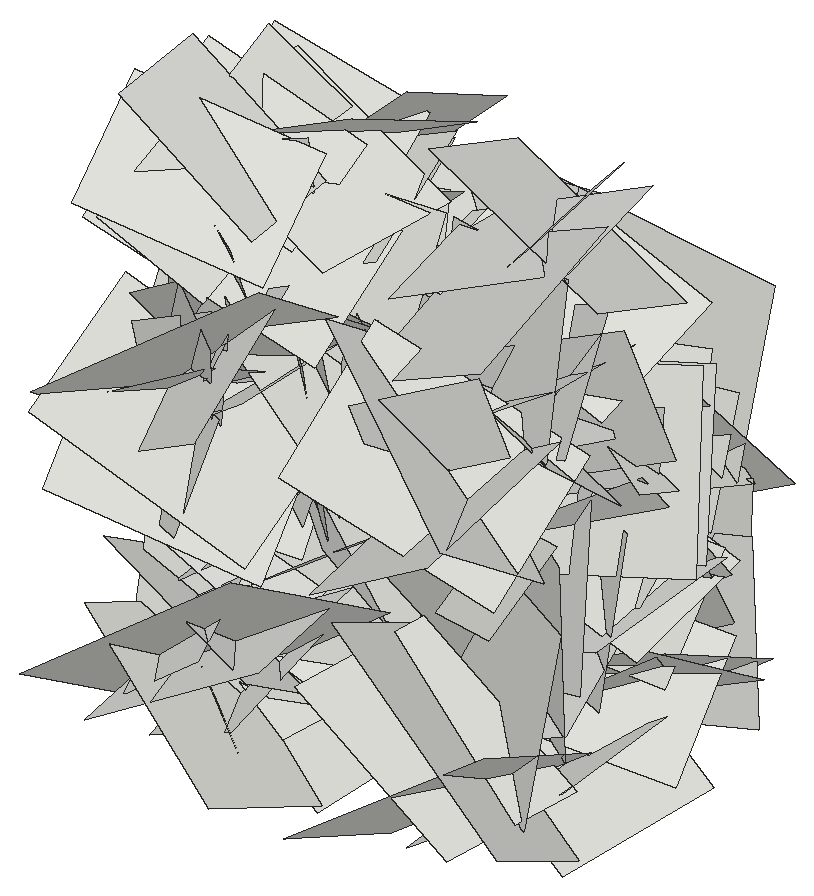
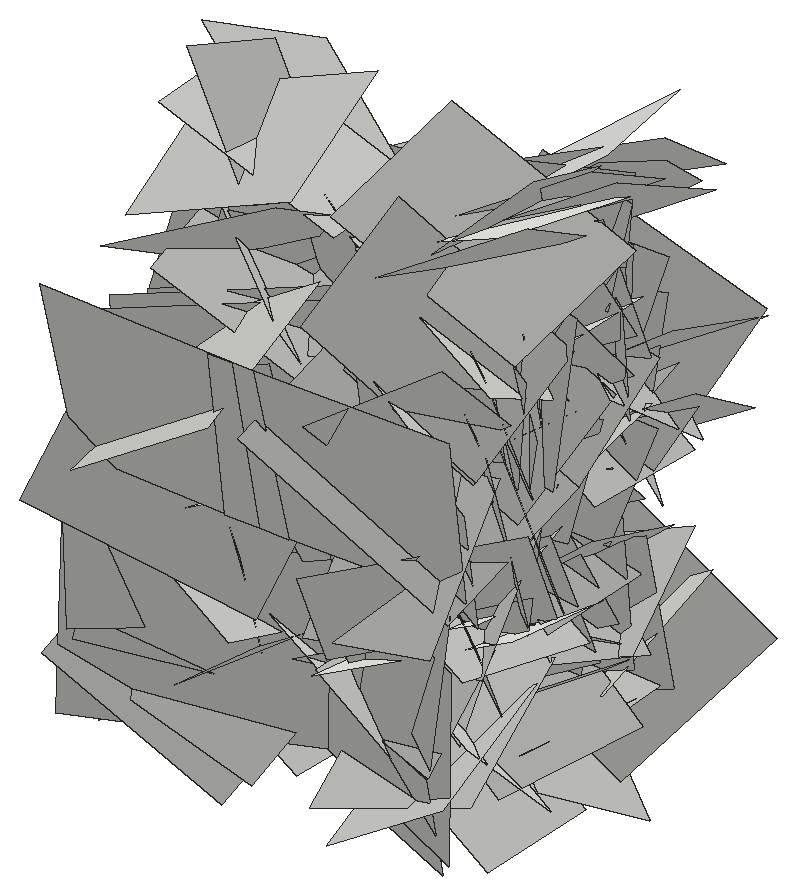
# SketchUp Ruby script. Lengths in inches.
U = 1.inch
M = Sketchup.active_model
def pt(a) = Geom::Point3d.new(a.map { |v| v * U })
def face(e, loops, mat)
  f = e.add_face(loops[0].map { |a| pt(a) })
  loops[1..].each { |l| e.add_face(l.map { |a| pt(a) }).erase! }
  f.material = f.back_material = mat if mat
  f
end
# faces: each face lists its corners as indices into pts; further lists are holes
def faces(e, pts, list, mat = nil) = list.each { |f| face(e, (f[0].is_a?(Array) ? f : [f]).map { |l| l.map { |i| pts[i] } }, mat) }
# xy, xz, yz: faces in a plane at the given z, y or x. An outline is a flat list of corners, or four numbers for a rectangle; further outlines are holes
def ring(l) = l.size == 4 ? [[l[0], l[1]], [l[2], l[1]], [l[2], l[3]], [l[0], l[3]]] : l.each_slice(2).to_a
def flat(e, list, mat, &to3) = list.each { |f| face(e, (f[0].is_a?(Array) ? f : [f]).map { |l| ring(l).map { |u, v| to3.(u, v) } }, mat) }
def xy(e, z, list, mat = nil) = flat(e, list, mat) { |x, y| [x, y, z] }
def xz(e, y, list, mat = nil) = flat(e, list, mat) { |x, z| [x, y, z] }
def yz(e, x, list, mat = nil) = flat(e, list, mat) { |y, z| [x, y, z] }
def lines(e, pts, list) = list.each { |a, b| e.add_line(pt(pts[a]), pt(pts[b])) }
# prism: a flat outline (further loops are holes) pulled along v
def prism(e, loops, v, mat = nil)
  f = face(e, loops, mat); d = Geom::Vector3d.new(v.map { |x| x * U })
  f.pushpull(f.normal.samedirection?(d) ? d.length : -d.length)
end
def box(e, o, s, mat = nil) = prism(e, [[o, [o[0] + s[0], o[1], o[2]], [o[0] + s[0], o[1] + s[1], o[2]], [o[0], o[1] + s[1], o[2]]]], [0, 0, s[2]], mat)
def at(x, y, z, deg = 0) = Geom::Transformation.translation(pt([x, y, z])) * Geom::Transformation.rotation(ORIGIN, Z_AXIS, deg.degrees)
def axes(o, x, y, z) = Geom::Transformation.new([*x, 0, *y, 0, *z, 0, *pt(o).to_a, 1])
def part(name) = M.definitions.add(name)
# library, detail: a bought-in or finely detailed component or shape, given as its bounding box
def library(name, o, s) = part(name).tap { |d| box(d.entities, o, s) }
def detail(e, o, s) = box(e.add_group.entities, o, s)
def put(e, d, t, mat = nil) = e.add_instance(d, t).tap { |i| i.material = mat if mat }
def group(e, t, mat = nil) = e.add_group.tap { |g| g.transformation = t; g.material = mat if mat }.entities
root = M.entities
c1 = part("Component\#6")
p = [[0.01,0,0],[0,3.24,4.54],[4.32,3.24,4.54],[4.33,0,0]]
faces(c1.entities,p,[[0,1,2,3]])
put(root,c1,axes([28.31,209.1,25.86],[0.06992,-0.92649,-0.30548],[0.11921,-0.29692,0.92479],[-1.02719,-0.09753,0.08653]))
put(root,c1,axes([24.34,209.1,25.86],[-0.06992,-0.92649,-0.30548],[-0.11921,-0.29692,0.92479],[1.02719,-0.09753,0.08653]))
put(root,c1,axes([24.34,210.17,27.25],[0.0389,-0.19659,0.74237],[0.03773,0.74285,0.19496],[0.81316,-0.02506,-0.04456]))
put(root,c1,axes([28.31,202.89,32.22],[0.0211,0.0618,0.84202],[0.01452,0.84212,-0.06213],[-0.89482,0.01512,0.01885]))
put(root,c1,axes([24.34,209.27,26.87],[0.02942,-0.98917,0.00062],[-0.2303,-0.00549,0.9654],[1.02292,0.02721,0.21733]))
put(root,c1,axes([24.34,208.86,27.22],[-0.22907,0.58895,0.94038],[-0.09031,0.94642,-0.61231],[1.17269,0.18793,0.13653]))
put(root,c1,axes([24.34,209.72,22.08],[-0.18138,-0.91546,-0.54155],[-0.07402,-0.53767,0.93095],[1.12504,-0.18297,-0.02606]))
put(root,c1,axes([24.34,200.125,30.08],[-0.25415,0.9144,0.59243],[-0.00684,0.60541,-0.93704],[1.1549,0.20481,0.12483]))
put(root,c1,axes([28.31,207.43,34.16],[-0.11276,0.04323,0.70746],[0.03845,0.71477,-0.03823],[-0.75032,0.03013,-0.10828]))
put(root,c1,axes([24.34,204.07,39.0625],[-0.02986,0.79051,0.40956],[0.00815,0.40997,-0.79076],[0.94369,0.02147,0.01979]))
put(root,c1,axes([28.31,209.14,33.82],[-0.16184,0.36707,0.52708],[0.01835,0.54392,-0.37378],[-0.68059,-0.07262,-0.13541]))
put(root,c1,axes([24.34,210.92,34.25],[0.13403,0.53039,0.57824],[-0.04314,0.58935,-0.53168],[0.83061,-0.05497,-0.12092]))
put(root,c1,axes([28.31,209.37,33.75],[0.00852,0.3462,-0.76666],[0.09329,-0.76284,-0.34355],[-0.88678,-0.07692,-0.04351]))
put(root,c1,axes([28.31,201.89,25.36],[-0.12511,0.60489,0.30184],[0.04372,0.31228,-0.60968],[-0.71524,-0.08672,-0.09007]))
put(root,c1,axes([24.34,206.58,28.49],[0.01093,-0.51913,0.63451],[0.10311,0.63085,0.51456],[0.86287,-0.06881,-0.06953]))
put(root,c1,axes([28.31,207.4,37.82],[0.14382,-0.92009,0.02073],[0.06912,0.03051,0.92748],[-0.97309,-0.13382,0.06894]))
put(root,c1,axes([28.31,211.91,37.97],[0.10192,-0.72839,-0.40458],[0.00784,-0.4065,0.73361],[-0.88316,-0.08767,-0.04018]))
put(root,c1,axes([28.31,205,37.54],[-0.1597,-0.46751,-0.41946],[0.05532,-0.43919,0.47075],[-0.66349,0.07592,0.14021]))
put(root,c1,axes([24.34,204.65,32.19],[0.14144,0.68446,-0.34907],[0.03425,-0.35898,-0.69154],[0.81371,-0.10387,0.08978]))
put(root,c1,axes([24.34,205.35,34.65],[0.12302,0.37909,0.72016],[-0.00858,0.72795,-0.38188],[0.86263,-0.04682,-0.1065]))
put(root,c1,axes([28.31,209.27,26.93],[-0.01951,-0.6006,0.29742],[-0.06663,0.29777,0.59742],[-0.70729,-0.01148,-0.06448]))
put(root,c1,axes([28.31,204.33,34.72],[0.02793,-0.28222,0.66343],[-0.05268,0.66158,0.28341],[-0.7624,-0.05605,0.00473]))
put(root,c1,axes([24.34,210.23,35.31],[0.06568,0.00099,-0.81141],[0.08224,-0.81005,0.00494],[0.85616,0.07773,0.06177]))
put(root,c1,axes([28.31,207.11,31.75],[0.23783,0.22127,0.93353],[0.03566,0.95632,-0.23476],[-1.01634,0.08533,0.21022]))
put(root,c1,axes([24.34,201.41,38.375],[-0.12316,0.77538,0.57304],[0.12545,0.58429,-0.76661],[1.01427,0.02189,0.1644]))
put(root,c1,axes([24.34,210.61,30.96],[0.02538,-1.03384,0.49264],[-0.2847,0.47394,1.00764],[1.18007,0.13657,0.23251]))
put(root,c1,axes([24.34,212.48,33.12],[0.02538,-1.03384,0.49264],[-0.2847,0.47394,1.00764],[1.18007,0.13657,0.23251]))
put(root,c1,axes([28.31,206.77,29.69],[-0.13468,0.0618,0.68245],[0.14259,0.68282,-0.03679],[-0.71222,0.12502,-0.13642]))
put(root,c1,axes([24.34,202.75,27.49],[-0.17368,0.85862,-0.51485],[0.1903,-0.48804,-0.87105],[1.04401,0.2318,0.07312]))
put(root,c1,axes([28.31,211.1,35.2],[-0.07899,0.5337,0.27791],[-0.02897,0.27674,-0.53878],[-0.63716,-0.07875,-0.00996]))
put(root,c1,axes([28.31,212.78,35.18],[0.06835,-0.19577,-0.64021],[-0.13077,-0.63563,0.18195],[-0.69749,0.09999,-0.09685]))
put(root,c1,axes([28.31,200.85,29.625],[0.04324,0.39016,0.69087],[0.10275,0.68414,-0.39209],[-0.83473,0.10443,-0.01247]))
put(root,c1,axes([28.31,202.23,33.91],[-0.02493,0.60398,0.49928],[0.17768,0.49182,-0.58706],[-0.81142,0.08914,-0.14389]))
put(root,c1,axes([28.31,204.22,36.67],[-0.08595,0.41822,-0.43473],[0.01861,-0.43682,-0.42351],[-0.63917,-0.06896,0.04613]))
put(root,c1,axes([28.31,206.625,39.5],[0.00312,0.09172,-0.66161],[-0.00201,-0.66161,-0.09173],[-0.70801,0.00228,-0.00265]))
put(root,c1,axes([28.31,212.36,26.625],[0.06935,-0.64087,-0.11796],[-0.11905,-0.12787,0.63241],[-0.68039,-0.04294,-0.12268]))
put(root,c1,axes([28.31,204.95,35.05],[-0.03568,0.1968,-0.61743],[0.04358,-0.61637,-0.1987],[-0.68554,-0.04943,0.01951]))
put(root,c1,axes([24.34,207.21,30.03],[-0.00943,-1.01637,-0.0193],[-0.00822,-0.01923,1.01638],[1.07752,-0.00904,0.00758]))
put(root,c1,axes([24.34,205.67,24.52],[0.15369,0.87531,0.08009],[-0.01982,0.08422,-0.88666],[0.9315,-0.14262,-0.03208]))
put(root,c1,axes([24.34,206.36,33.23],[-0.09168,1.1059,0.20164],[-0.04784,0.19866,-1.1089],[1.19063,0.09314,-0.02903]))
put(root,c1,axes([24.34,211.47,22.62],[-0.20513,-1.22241,0.07319],[-0.04122,0.08019,1.23659],[1.29742,-0.19072,0.05085]))
put(root,c1,axes([28.31,202.42,34.22],[0.03507,0.56649,-0.26791],[-0.06705,-0.26389,-0.56581],[-0.66085,0.05684,0.04319]))
put(root,c1,axes([28.31,203.96,20.97],[-0.02025,-0.24988,0.58047],[0.03388,0.57961,0.25056],[-0.66903,0.03691,-0.00488]))
put(root,c1,axes([28.31,208.95,27.68],[0.1117,0.11156,-0.75397],[0.06454,-0.75994,-0.10393],[-0.80532,-0.04543,-0.11291]))
put(root,c1,axes([28.31,211.4,20.36],[0.11841,0.02386,0.67628],[-0.07272,0.6823,-0.01274],[-0.7136,-0.06557,0.11352]))
put(root,c1,axes([24.34,209.77,25.57],[-0.04769,1.02209,-0.46416],[-0.05126,-0.46587,-1.02116],[1.18879,0.02092,-0.06265]))
put(root,c1,axes([24.34,212.41,27.7],[0.11035,-0.46639,-0.85158],[-0.0233,-0.85737,0.46687],[1.02892,0.03061,0.1019]))
put(root,c1,axes([28.31,210.37,37.54],[0.0852,-0.7988,-0.26142],[0.21653,-0.23617,0.78446],[-0.8642,-0.13792,0.17078]))
put(root,c1,axes([28.31,207.84,29.22],[0.13906,-0.51177,-0.49755],[-0.00544,-0.50655,0.51967],[-0.75658,-0.09042,-0.09518]))
put(root,c1,axes([24.34,211.63,27.44],[0.13698,0.50835,-0.7639],[0.02564,-0.77306,-0.51036],[0.97231,-0.05123,0.12108]))
put(root,c1,axes([24.34,212.85,24.81],[-0.10314,-0.72888,-0.73382],[0.20394,-0.73695,0.70648],[1.07722,0.06973,-0.20401]))
put(root,c1,axes([24.34,211.43,33.78],[-0.23599,-0.36182,-1.29322],[-0.09706,-1.30373,0.38052],[1.42014,-0.14923,-0.18889]))
put(root,c1,axes([24.34,199.54,32.72],[-0.14681,1.15124,0.44909],[-0.05729,0.44582,-1.15954],[1.30862,0.14867,-0.00039]))
put(root,c1,axes([24.34,206.07,20.81],[-0.31441,-1.20333,0.63493],[-0.01893,0.65323,1.22967],[1.44208,-0.25378,0.15457]))
put(root,c1,axes([24.34,208.01,36.375],[-0.10923,0.38133,-1.06486],[0.05778,-1.06635,-0.38714],[1.19755,0.08623,-0.07845]))
put(root,c1,axes([24.34,212.99,32.26],[0.05541,-0.21084,-0.92918],[0.15034,-0.91849,0.21639],[0.99872,0.14996,0.01898]))
put(root,c1,axes([24.34,205.46,33.43],[0.14097,0.63084,0.7943],[-0.06243,0.80455,-0.62912],[1.07339,-0.03606,-0.14091]))
put(root,c1,axes([24.34,207.91,30.98],[-0.03881,-0.77727,0.6188],[0.26695,0.59174,0.75817],[1.01873,-0.18467,-0.1751]))
put(root,c1,axes([28.31,206,31.6],[0.1462,-0.08624,0.716],[0.07336,0.72719,0.07426],[-0.76092,0.05354,0.14472]))
put(root,c1,axes([28.31,210.56,30.82],[0.08988,0.23539,0.56706],[-0.00516,0.57268,-0.23699],[-0.65079,0.02797,0.0802]))
put(root,c1,axes([24.34,206.55,33.15],[0.00164,-0.95203,-0.71322],[-0.09471,-0.7113,0.94927],[1.25737,-0.05234,0.07244]))
put(root,c1,axes([24.34,206.8125,26.89],[-0.15204,1.11982,0.24611],[0.19339,0.26716,-1.10927],[1.19986,0.09884,0.20998]))
put(root,c1,axes([24.34,211.99,33.59],[-0.13241,-0.25962,-1.28668],[-0.09489,-1.2878,0.26854],[1.38813,-0.1128,-0.10438]))
put(root,c1,axes([24.34,206.95,24.98],[0.09414,0.39654,1.07266],[-0.12922,1.07305,-0.38659],[1.20532,0.08407,-0.12522]))
put(root,c1,axes([28.31,202.49,32.61],[0.11645,-0.17214,0.59947],[0.01233,0.60916,0.17278],[-0.661,-0.01896,0.10883]))
put(root,c1,axes([24.34,205.38,23.16],[0.04798,1.09948,0.05597],[0.01409,0.05547,-1.10036],[1.16688,-0.04588,0.01099]))
put(root,c1,axes([24.34,210.75,36.02],[-0.14272,-1.0645,0.43866],[0.22696,0.41079,1.0626],[1.19913,-0.20445,-0.14891]))
put(root,c1,axes([24.34,208.81,31.45],[-0.04602,0.84125,-1.04893],[-0.18208,-1.04435,-0.83047],[1.4136,-0.10713,-0.14111]))
put(root,c1,axes([24.34,213.59,29.33],[0.10669,0.07311,-1.12569],[-0.06812,-1.12796,-0.079],[1.19381,-0.0709,0.09609]))
put(root,c1,axes([24.34,201.95,25.76],[0.02109,1.10253,-0.4508],[-0.04504,-0.44992,-1.10225],[1.2618,-0.03449,-0.03181]))
put(root,c1,axes([24.34,213.06,27.02],[-0.109,-1.16412,-0.17966],[0.1638,-0.19212,1.15639],[1.23778,-0.07709,-0.16885]))
put(root,c1,axes([24.34,201.85,37.73],[-0.10519,1.13817,0.58904],[-0.00109,0.59073,-1.14161],[1.35845,0.08861,0.0447]))
put(root,c1,axes([24.34,204.59,30.02],[-0.04301,-1.09683,0.72238],[-0.12053,0.72294,1.0913],[1.38692,0.02882,0.11724]))
put(root,c1,axes([24.34,209.74,33.23],[0.15201,0.07034,-1.21602],[-0.20156,-1.20811,-0.09231],[1.2753,-0.19933,0.13035]))
put(root,c1,axes([24.34,208.94,26.04],[-0.1299,1.02121,-0.60997],[0.25035,-0.5801,-1.01865],[1.23578,0.22487,0.14225]))
put(root,c1,axes([24.34,213.71,29.11],[-0.07729,-1.24842,0.49404],[-0.03127,0.49613,1.24937],[1.42283,-0.05691,0.0543]))
put(root,c1,axes([24.34,211.375,32.78],[-0.08242,0.8278,-0.94283],[0.12426,-0.93571,-0.83122],[1.32412,0.13934,0.01932]))
put(root,c1,axes([24.34,211.85,35.53],[0.11979,-0.95717,-0.48165],[0.13908,-0.46832,0.96146],[1.12727,0.15949,-0.06744]))
put(root,c1,axes([24.34,203.71,22.72],[-0.0324,0.32539,1.27516],[0.00551,1.27553,-0.32536],[1.39498,0.00251,0.0309]))
put(root,c1,axes([24.34,205.99,22.98],[0.14358,-1.11124,-0.06865],[0.09474,-0.05808,1.11649],[1.17635,0.14031,-0.08154]))
put(root,c1,axes([24.34,205.63,39.17],[0.17317,1.06099,0.10432],[0.22006,0.07185,-1.05594],[1.10844,-0.18002,0.19334]))
put(root,c1,axes([24.34,205.46,24.09],[0.08024,0.04196,1.34674],[-0.06239,1.34768,-0.03868],[1.42687,0.05657,-0.07742]))
put(root,c1,axes([24.34,204.65,33.57],[0.11682,0.36237,1.1463],[0.15256,1.13885,-0.37385],[1.26518,-0.17079,-0.06076]))
put(root,c1,axes([24.34,211.92,20.51],[0.20622,-1.25394,-0.15944],[-0.06822,-0.17093,1.26581],[1.33814,0.18453,0.0891]))
put(root,c1,axes([24.34,213.57,27.56],[-0.01798,0.03957,-1.39555],[0.22262,-1.3797,-0.04168],[1.46303,0.21042,-0.01081]))
put(root,c1,axes([24.34,205.51,24.88],[0.13882,1.11155,0.63897],[0.19603,0.6192,-1.11507],[1.34484,-0.205,0.09658]))
put(root,c1,axes([23.99,214.11,35.21],[0.07772,-0.27644,-1.33377],[0.91911,-1.02064,0.2592],[1.11351,0.86175,-0.12086]))
put(root,c1,axes([24.34,205.05,35.75],[0.23328,1.34713,-0.22992],[0.05022,-0.24027,-1.36238],[1.44774,-0.20874,0.08431]))
put(root,c1,axes([24.34,206.12,25.83],[0.28838,0.48251,1.20317],[0.13396,1.21365,-0.51529],[1.36755,-0.22063,-0.20324]))
put(root,c1,axes([38.11,206.12,25.83],[-0.28838,0.48251,1.20317],[-0.13396,1.21365,-0.51529],[-1.36755,-0.22063,-0.20324]))
put(root,c1,axes([38.11,205.05,35.75],[-0.23328,1.34713,-0.22992],[-0.05022,-0.24027,-1.36238],[-1.44774,-0.20874,0.08431]))
put(root,c1,axes([38.46,214.11,35.21],[-0.07772,-0.27644,-1.33377],[-0.91911,-1.02064,0.2592],[-1.11351,0.86175,-0.12086]))
put(root,c1,axes([38.11,205.51,24.88],[-0.13882,1.11155,0.63897],[-0.19603,0.6192,-1.11507],[-1.34484,-0.205,0.09658]))
put(root,c1,axes([38.11,213.57,27.56],[0.01798,0.03957,-1.39555],[-0.22262,-1.3797,-0.04168],[-1.46303,0.21042,-0.01081]))
put(root,c1,axes([38.11,211.92,20.51],[-0.20622,-1.25394,-0.15944],[0.06822,-0.17093,1.26581],[-1.33814,0.18453,0.0891]))
put(root,c1,axes([38.11,204.65,33.57],[-0.11682,0.36237,1.1463],[-0.15256,1.13885,-0.37385],[-1.26518,-0.17079,-0.06076]))
put(root,c1,axes([38.11,205.46,24.09],[-0.08024,0.04196,1.34674],[0.06239,1.34768,-0.03868],[-1.42687,0.05657,-0.07742]))
put(root,c1,axes([38.11,205.63,39.17],[-0.17317,1.06099,0.10432],[-0.22006,0.07185,-1.05594],[-1.10844,-0.18002,0.19334]))
put(root,c1,axes([38.11,205.99,22.98],[-0.14358,-1.11124,-0.06865],[-0.09474,-0.05808,1.11649],[-1.17635,0.14031,-0.08154]))
put(root,c1,axes([38.11,203.71,22.72],[0.0324,0.32539,1.27516],[-0.00551,1.27553,-0.32536],[-1.39498,0.00251,0.0309]))
put(root,c1,axes([38.11,211.85,35.53],[-0.11979,-0.95717,-0.48165],[-0.13908,-0.46832,0.96146],[-1.12727,0.15949,-0.06744]))
put(root,c1,axes([38.11,211.375,32.78],[0.08242,0.8278,-0.94283],[-0.12426,-0.93571,-0.83122],[-1.32412,0.13934,0.01932]))
put(root,c1,axes([38.11,213.71,29.11],[0.07729,-1.24842,0.49404],[0.03127,0.49613,1.24937],[-1.42283,-0.05691,0.0543]))
put(root,c1,axes([38.11,208.94,26.04],[0.1299,1.02121,-0.60997],[-0.25035,-0.5801,-1.01865],[-1.23578,0.22487,0.14225]))
put(root,c1,axes([38.11,209.74,33.23],[-0.15201,0.07034,-1.21602],[0.20156,-1.20811,-0.09231],[-1.2753,-0.19933,0.13035]))
put(root,c1,axes([38.11,204.59,30.02],[0.04301,-1.09683,0.72238],[0.12053,0.72294,1.0913],[-1.38692,0.02882,0.11724]))
put(root,c1,axes([38.11,201.85,37.73],[0.10519,1.13817,0.58904],[0.00109,0.59073,-1.14161],[-1.35845,0.08861,0.0447]))
put(root,c1,axes([38.11,213.06,27.02],[0.109,-1.16412,-0.17966],[-0.1638,-0.19212,1.15639],[-1.23778,-0.07709,-0.16885]))
put(root,c1,axes([38.11,201.95,25.76],[-0.02109,1.10253,-0.4508],[0.04504,-0.44992,-1.10225],[-1.2618,-0.03449,-0.03181]))
put(root,c1,axes([38.11,213.59,29.33],[-0.10669,0.07311,-1.12569],[0.06812,-1.12796,-0.079],[-1.19381,-0.0709,0.09609]))
put(root,c1,axes([38.11,208.81,31.45],[0.04602,0.84125,-1.04893],[0.18208,-1.04435,-0.83047],[-1.4136,-0.10713,-0.14111]))
put(root,c1,axes([38.11,210.75,36.02],[0.14272,-1.0645,0.43866],[-0.22696,0.41079,1.0626],[-1.19913,-0.20445,-0.14891]))
put(root,c1,axes([38.11,205.38,23.16],[-0.04798,1.09948,0.05597],[-0.01409,0.05547,-1.10036],[-1.16688,-0.04588,0.01099]))
put(root,c1,axes([34.14,202.49,32.61],[-0.11645,-0.17214,0.59947],[-0.01233,0.60916,0.17278],[0.661,-0.01896,0.10883]))
put(root,c1,axes([38.11,206.95,24.98],[-0.09414,0.39654,1.07266],[0.12922,1.07305,-0.38659],[-1.20532,0.08407,-0.12522]))
put(root,c1,axes([38.11,211.99,33.59],[0.13241,-0.25962,-1.28668],[0.09489,-1.2878,0.26854],[-1.38813,-0.1128,-0.10438]))
put(root,c1,axes([38.11,206.8125,26.89],[0.15204,1.11982,0.24611],[-0.19339,0.26716,-1.10927],[-1.19986,0.09884,0.20998]))
put(root,c1,axes([38.11,206.55,33.15],[-0.00164,-0.95203,-0.71322],[0.09471,-0.7113,0.94927],[-1.25737,-0.05234,0.07244]))
put(root,c1,axes([34.14,210.56,30.82],[-0.08988,0.23539,0.56706],[0.00516,0.57268,-0.23699],[0.65079,0.02797,0.0802]))
put(root,c1,axes([34.14,206,31.6],[-0.1462,-0.08624,0.716],[-0.07336,0.72719,0.07426],[0.76092,0.05354,0.14472]))
put(root,c1,axes([38.11,207.91,30.98],[0.03881,-0.77727,0.6188],[-0.26695,0.59174,0.75817],[-1.01873,-0.18467,-0.1751]))
put(root,c1,axes([38.11,205.46,33.43],[-0.14097,0.63084,0.7943],[0.06243,0.80455,-0.62912],[-1.07339,-0.03606,-0.14091]))
put(root,c1,axes([38.11,212.99,32.26],[-0.05541,-0.21084,-0.92918],[-0.15034,-0.91849,0.21639],[-0.99872,0.14996,0.01898]))
put(root,c1,axes([38.11,208.01,36.375],[0.10923,0.38133,-1.06486],[-0.05778,-1.06635,-0.38714],[-1.19755,0.08623,-0.07845]))
put(root,c1,axes([38.11,206.07,20.81],[0.31441,-1.20333,0.63493],[0.01893,0.65323,1.22967],[-1.44208,-0.25378,0.15457]))
put(root,c1,axes([38.11,199.54,32.72],[0.14681,1.15124,0.44909],[0.05729,0.44582,-1.15954],[-1.30862,0.14867,-0.00039]))
put(root,c1,axes([38.11,211.43,33.78],[0.23599,-0.36182,-1.29322],[0.09706,-1.30373,0.38052],[-1.42014,-0.14923,-0.18889]))
put(root,c1,axes([38.11,212.85,24.81],[0.10314,-0.72888,-0.73382],[-0.20394,-0.73695,0.70648],[-1.07722,0.06973,-0.20401]))
put(root,c1,axes([38.11,211.63,27.44],[-0.13698,0.50835,-0.7639],[-0.02564,-0.77306,-0.51036],[-0.97231,-0.05123,0.12108]))
put(root,c1,axes([34.14,207.84,29.22],[-0.13906,-0.51177,-0.49755],[0.00544,-0.50655,0.51967],[0.75658,-0.09042,-0.09518]))
put(root,c1,axes([34.14,210.37,37.54],[-0.0852,-0.7988,-0.26142],[-0.21653,-0.23617,0.78446],[0.8642,-0.13792,0.17078]))
put(root,c1,axes([38.11,212.41,27.7],[-0.11035,-0.46639,-0.85158],[0.0233,-0.85737,0.46687],[-1.02892,0.03061,0.1019]))
put(root,c1,axes([38.11,209.77,25.57],[0.04769,1.02209,-0.46416],[0.05126,-0.46587,-1.02116],[-1.18879,0.02092,-0.06265]))
